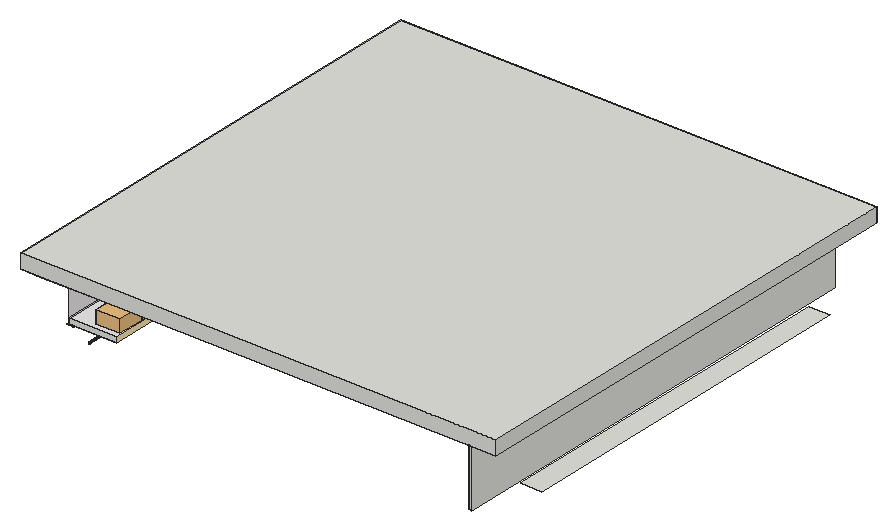
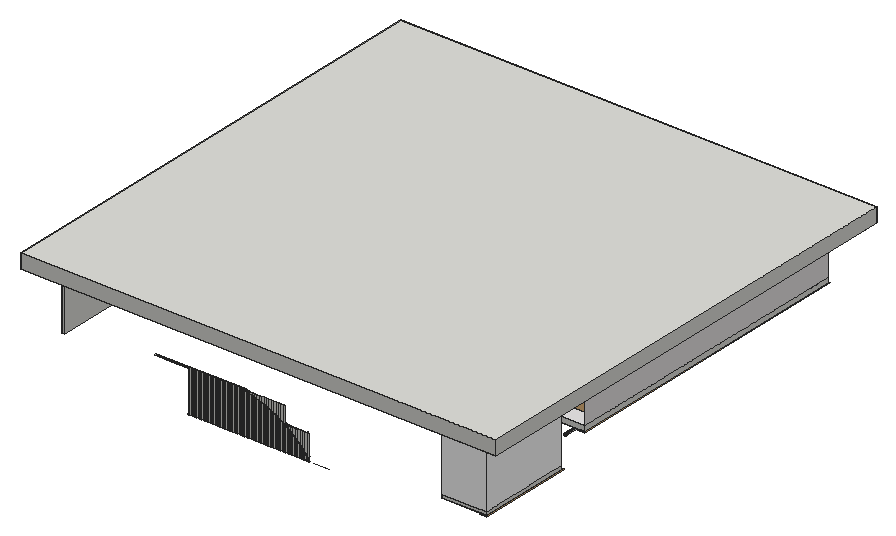
# SketchUp Ruby script. Lengths in inches.
U = 1.inch
M = Sketchup.active_model
def pt(a) = Geom::Point3d.new(a.map { |v| v * U })
def face(e, loops, mat)
  f = e.add_face(loops[0].map { |a| pt(a) })
  loops[1..].each { |l| e.add_face(l.map { |a| pt(a) }).erase! }
  f.material = f.back_material = mat if mat
  f
end
# faces: each face lists its corners as indices into pts; further lists are holes
def faces(e, pts, list, mat = nil) = list.each { |f| face(e, (f[0].is_a?(Array) ? f : [f]).map { |l| l.map { |i| pts[i] } }, mat) }
# xy, xz, yz: faces in a plane at the given z, y or x. An outline is a flat list of corners, or four numbers for a rectangle; further outlines are holes
def ring(l) = l.size == 4 ? [[l[0], l[1]], [l[2], l[1]], [l[2], l[3]], [l[0], l[3]]] : l.each_slice(2).to_a
def flat(e, list, mat, &to3) = list.each { |f| face(e, (f[0].is_a?(Array) ? f : [f]).map { |l| ring(l).map { |u, v| to3.(u, v) } }, mat) }
def xy(e, z, list, mat = nil) = flat(e, list, mat) { |x, y| [x, y, z] }
def xz(e, y, list, mat = nil) = flat(e, list, mat) { |x, z| [x, y, z] }
def yz(e, x, list, mat = nil) = flat(e, list, mat) { |y, z| [x, y, z] }
def lines(e, pts, list) = list.each { |a, b| e.add_line(pt(pts[a]), pt(pts[b])) }
# prism: a flat outline (further loops are holes) pulled along v
def prism(e, loops, v, mat = nil)
  f = face(e, loops, mat); d = Geom::Vector3d.new(v.map { |x| x * U })
  f.pushpull(f.normal.samedirection?(d) ? d.length : -d.length)
end
def box(e, o, s, mat = nil) = prism(e, [[o, [o[0] + s[0], o[1], o[2]], [o[0] + s[0], o[1] + s[1], o[2]], [o[0], o[1] + s[1], o[2]]]], [0, 0, s[2]], mat)
def at(x, y, z, deg = 0) = Geom::Transformation.translation(pt([x, y, z])) * Geom::Transformation.rotation(ORIGIN, Z_AXIS, deg.degrees)
def axes(o, x, y, z) = Geom::Transformation.new([*x, 0, *y, 0, *z, 0, *pt(o).to_a, 1])
def part(name) = M.definitions.add(name)
# library, detail: a bought-in or finely detailed component or shape, given as its bounding box
def library(name, o, s) = part(name).tap { |d| box(d.entities, o, s) }
def detail(e, o, s) = box(e.add_group.entities, o, s)
def put(e, d, t, mat = nil) = e.add_instance(d, t).tap { |i| i.material = mat if mat }
def group(e, t, mat = nil) = e.add_group.tap { |g| g.transformation = t; g.material = mat if mat }.entities
root = M.entities
M.materials.add("Generic").color = [234, 232, 232]
M.materials.add("Gold 10k").color = [251, 232, 180]
M.materials.add("[Color M00]").color = [255, 255, 255]
M.materials.add("[Color M07]").color = [58, 58, 58]
c1 = library("Group\#3",[-0.5,-0.5,-0.1],[3,40,0.2])
c2 = library("Armillary Sphere 37-31",[-7.11,-7.1,0],[14.21,14.18,18.13])
c3 = library("Decorative Deer 209 004",[-1.58,-4.16,0],[3.36,7.25,10.63])
c4 = library("Group\#5",[-0.5,-0.5,-0.1],[3,127.16,0.2])
c5 = library("Clothes 159 005",[-5.11,-5.34,0.03],[10.26,10.67,5.26])
c6 = library("Air Conditioning 001",[-17.62,-7.68,0],[35.24,7.68,11.77])
c7 = library("Fan 90-20",[-15.86,-15.86,-9.19],[31.73,31.72,9.19])
c8 = library("Group\#2",[-0.5,-0.5,-0.1],[3,40,0.2])
c9 = library("Group\#6",[-0.5,-0.5,-0.1],[3,127.16,0.2])
c10 = library("Tlon Light 1950 Ceiling 152 010",[-38.39,-38.39,-3.78],[76.78,76.78,3.41])
c11 = library("Group\#13",[-0.5,-0.5,0],[56.22,1,2.75])
c12 = library("Group\#14",[-0.5,-0.5,0],[1,91.6,2.75])
c13 = library("Group\#15",[-0.5,-0.5,0],[1,91.6,2.75])
c14 = library("Group\#10",[-0.5,-0.5,0],[95.14,130.51,2.5625])
c15 = library("Group\#11",[-0.5,-0.5,0],[127.98,1,2.5625])
c16 = library("Group\#12",[-0.5,-0.5,0],[1,163.35,2.5625])
c17 = library("Group\#16",[-0.5,-0.5,0],[1,164.23,2.5625])
c18 = library("Group\#17",[-0.5,-0.5,0],[127.98,1,2.5625])
xy(root,84.67,[[86.13,189.625,86.28,189.875],[86.875,189.625,87.28,189.875],[87.875,189.625,88.28,189.875],[88.875,189.625,89.28,189.875],[89.875,189.625,90.28,189.875],
  [90.875,189.625,91.28,189.875],[91.875,189.625,92.28,189.875],[92.875,189.625,93.28,189.875],[93.875,189.625,94.28,189.875],[94.875,189.625,95.28,189.875],
  [95.875,189.625,96.28,189.875],[96.875,189.625,97.28,189.875],[97.875,189.625,98.28,189.875],[98.875,189.625,99.28,189.875],[99.875,189.625,100.28,189.875],
  [100.875,189.625,101.28,189.875],[101.875,189.625,102.28,189.875],[102.875,189.625,103.28,189.875],[103.875,189.625,104.28,189.875],[104.875,189.625,105.28,189.875],
  [105.875,189.625,106.28,189.875],[106.875,189.625,107.28,189.875],[107.875,189.625,108.28,189.875],[108.875,189.625,109.28,189.875],[109.875,189.625,110.28,189.875],
  [110.875,189.625,111.28,189.875],[111.875,189.625,112.28,189.875],[112.875,189.625,113.28,189.875],[113.875,189.625,114.28,189.875],[114.875,189.625,115.28,189.875],
  [115.875,189.625,116.28,189.875],[116.875,189.625,117.28,189.875],[117.875,189.625,118.28,189.875],[118.875,189.625,119.28,189.875],[119.875,189.625,120.28,189.875],
  [120.875,189.625,121.28,189.875],[121.875,189.625,122.28,189.875],[122.875,189.625,123.28,189.875],[123.875,189.625,124.28,189.875],[124.875,189.625,125.28,189.875],
  [125.875,189.625,126.28,189.875],[126.875,189.625,127.28,189.875],[127.875,189.625,128.28,189.875],[128.875,189.625,129.28,189.875],[129.875,189.625,130.28,189.875],
  [130.875,189.625,131.28,189.875],[131.875,189.625,132.28,189.875],[132.875,189.625,133.28,189.875],[133.875,189.625,134.28,189.875],[134.28,189.625,134.75,189.875],
  [83.86,189.8125,83.93,189.875],[84.28,189.8125,84.49,189.875],[84.875,189.8125,85.09,189.875],[85.28,189.8125,85.66,189.875],[85.875,189.8125,85.92,189.875],
  [85.92,189.8125,86.04,189.875],[86.04,189.8125,86.13,189.875]])
xy(root,86.88,[[16.5,145.84,33,184.83]])
xy(root,88.09,[[14.5,145.84,33,184.83]],"[Color M00]")
xy(root,96,[[186.625,0,187.95,189],[189,24,198,174]])
xy(root,98.59,[[13.1875,11.43,31,137.59]],"Generic")
xy(root,100.64,[[11.1875,11.43,31,137.59]],"Generic")
xy(root,101.92,[[112.34,189,112.34,189.625,112.875,189.625,112.875,189.875,113.28,189.875,113.28,189.625,113.875,189.625,113.875,189.875,114.28,189.875,114.28,189.625,114.875,189.625,114.875,189.875,115.28,189.875,115.28,189.625,115.875,189.625,115.875,189.875,116.28,189.875,116.28,189.625,116.875,189.625,116.875,189.875,117.28,189.875,117.28,189.625,117.875,189.625,117.875,189.875,118.28,189.875,118.28,189.625,118.875,189.625,118.875,189.875,119.28,189.875,119.28,189.625,119.875,189.625,119.875,189.875,120.28,189.875,120.28,189.625,120.875,189.625,120.875,189.875,121.28,189.875,121.28,189.625,121.875,189.625,121.875,189.875,122.28,189.875,122.28,189.625,122.875,189.625,122.875,189.875,123.28,189.875,123.28,189.625,123.875,189.625,123.875,189.875,124.28,189.875,124.28,189.625,124.875,189.625,124.875,189.875,125.28,189.875,125.28,189.625,125.875,189.625,125.875,189.875,126.28,189.875,126.28,189.625,126.875,189.625,126.875,189.875,127.28,189.875,127.28,189.625,127.875,189.625,127.875,189.875,128.28,189.875,128.28,189.625,128.875,189.625,128.875,189.875,129.28,189.875,129.28,189.625,129.875,189.625,129.875,189.875,130.28,189.875,130.28,189.625,130.875,189.625,130.875,189.875,131.28,189.875,131.28,189.625,131.875,189.625,131.875,189.875,132.28,189.875,132.28,189.625,132.875,189.625,132.875,189.875,133.28,189.875,133.28,189.625,133.875,189.625,133.875,189.875,134.28,189.875,134.28,189.625,134.875,189.625,134.875,189.875,135.28,189.875,135.28,189.75,135.875,189.75,135.875,189.875,136.28,189.875,136.28,189.75,136.875,189.75,136.875,189.875,137.28,189.875,137.28,189.75,137.875,189.75,137.875,189.875,138.28,189.875,138.28,189.75,138.875,189.75,138.875,189.875,139.28,189.875,139.28,189.75,139.875,189.75,139.875,189.875,140.28,189.875,140.28,189.75,140.875,189.75,140.875,189.875,141.28,189.875,141.28,189.75,141.875,189.75,141.875,189.875,142.28,189.875,142.28,189.75,142.875,189.75,142.875,189.875,143.28,189.875,143.28,189.75,143.875,189.75,143.875,189.875,144.28,189.875,144.28,189.75,144.875,189.75,144.875,189.875,145.28,189.875,145.28,189.75,145.875,189.75,145.875,189.875,146.28,189.875,146.28,189.75,146.875,189.75,146.875,189.875,147.28,189.875,147.28,189.75,147.875,189.75,147.875,189.875,148.625,189.875,148.625,189],[134.28,189.625,134.875,189.875],[135.28,189.75,135.875,189.875],[136.28,189.75,136.875,189.875],[137.28,189.75,137.875,189.875],
  [138.28,189.75,138.875,189.875],[139.28,189.75,139.875,189.875],[140.28,189.75,140.875,189.875],[141.28,189.75,141.875,189.875],[142.28,189.75,142.875,189.875],
  [143.28,189.75,143.875,189.875],[144.28,189.75,144.875,189.875],[145.28,189.75,145.875,189.875],[146.28,189.75,146.875,189.875],[147.28,189.75,147.875,189.875]])
xy(root,114.93,[[33,52.82,34.4375,53.82],[34.4375,52.82,34.8125,53.82],[33,95.21,34.4375,96.21],[34.4375,95.21,34.8125,96.21]])
xy(root,114.93,[[33,12.43,34.4375,52.82],[34.4375,12.43,34.8125,52.82],[33,53.82,34.4375,95.21],[34.4375,53.82,34.8125,95.21],[33,96.21,34.4375,136.59],
  [34.4375,96.21,34.8125,136.59]],"[Color M07]")
xy(root,115.83,[[16.5,145.84,33,184.83]])
xy(root,115.93,[[13.1875,11.43,33,137.59]],"Generic")
xy(root,115.93,[[33,11.43,33.4375,12.43],[33.4375,11.43,34.4375,12.43],[34.4375,11.43,34.8125,12.43],[33,12.43,33.4375,136.59],[33.4375,12.43,34.4375,136.59],
  [34.4375,12.43,34.8125,136.59],[33,136.59,33.4375,137.59],[33.4375,136.59,34.4375,137.59],[34.4375,136.59,34.8125,137.59]],"[Color M07]")
xy(root,117.25,[[82.2,49.2,137.43,139.8]])
xy(root,118.7,[[70.35,189,151.87,189.875]])
xy(root,120,[[0,0,0,198,198,198,198,0,189,0,189,189,173.42,189,173.42,190.5,171.08,190.5,171.08,189,153.17,189,153.17,189.875,69.06,189.875,69.06,189,9,189,9,0],[9,0,33,7.36],[[33,0,33,189,69.06,189,69.06,189.875,153.17,189.875,153.17,189,171.08,189,171.08,190.5,173.42,190.5,173.42,189,186.625,189,186.625,0],[46.32,13.32,173.3,176.55]],[186.625,0,187.95,189],[187.95,0,189,189],
  [9,7.36,33,141.67],[9,7.36,33,189],[[62.75,29.75,156.88,159.25],[82.2,49.2,137.43,139.8]],[9,141.67,33,189]])
xy(root,122.5625,[[[46.32,13.32,173.3,176.55],[62.75,29.75,156.88,159.25]]])
xy(root,126,[[0,0,198,198]])
xz(root,0,[[186.625,96,187.95,120],[0,120,198,126]])
xz(root,11.43,[[11.1875,98.59,31,100.64]])
xz(root,12.43,[[33,114.93,34.4375,115.93],[34.4375,114.93,34.8125,115.93]])
xz(root,136.59,[[33,114.93,34.4375,115.93],[34.4375,114.93,34.8125,115.93]])
xz(root,137.59,[[19.57,94.12,19.47,94.13,19.37,94.17,19.29,94.23,19.23,94.32,19.1875,94.41,19.17,94.52,19.1875,94.62,19.23,94.72,19.29,94.8,19.37,94.86,19.47,94.9,19.57,94.92,19.68,94.9,19.77,94.86,19.86,94.8,19.92,94.72,19.96,94.62,19.97,94.52,19.96,94.41,19.92,94.32,19.86,94.23,19.77,94.17,19.68,94.13],[11.1875,98.59,31,100.64]])
xz(root,139.8,[[82.2,117.25,137.43,120]])
xz(root,145.84,[[14.5,86.88,33,88.09],[14.5,88.09,33,115.83]])
xz(root,159.25,[[123.42,120,156.88,122.5625]])
xz(root,184.83,[[14.5,86.88,33,88.09]])
xz(root,184.83,[[14.5,88.09,33,115.83]],"[Color M00]")
xz(root,189,[[186.625,96,187.95,120]])
xz(root,189.625,[[86.28,84.67,86.875,84.67,86.875,88.4,86.28,87.7],[87.28,84.67,87.875,84.67,87.875,89.52,87.68,89.33,87.28,88.86],[88.28,84.67,88.875,84.67,88.875,90.45,88.28,89.89],[89.28,84.67,89.875,84.67,89.875,91.375,89.28,90.82],[90.28,84.67,90.875,84.67,90.875,92.31,90.28,91.75],
  [91.28,84.67,91.875,84.67,91.875,93.09,91.28,92.65],[92.28,84.67,92.875,84.67,92.875,93.84,92.28,93.39],[93.28,84.67,93.875,84.67,93.875,94.58,93.28,94.13],[94.28,84.67,94.875,84.67,94.875,95.32,94.28,94.875],[95.28,84.67,95.875,84.67,95.875,95.91,95.28,95.56],
  [96.28,84.67,96.875,84.67,96.875,96.49,96.28,96.14],[97.28,84.67,97.875,84.67,97.875,97.07,97.28,96.72],[98.28,84.67,98.875,84.67,98.875,97.65,98.28,97.31],[99.28,84.67,99.875,84.67,99.875,98.11,99.28,97.84],[100.28,84.67,100.875,84.67,100.875,98.55,100.28,98.28],
  [101.28,84.67,101.875,84.67,101.875,98.99,101.28,98.73],[102.28,84.67,102.875,84.67,102.875,99.43,102.28,99.17],[103.28,84.67,103.875,84.67,103.875,99.8,103.28,99.61],[104.28,84.67,104.875,84.67,104.875,100.11,104.28,99.92],[105.28,84.67,105.875,84.67,105.875,100.43,105.28,100.24],
  [106.28,84.67,106.875,84.67,106.875,100.74,106.28,100.55],[107.28,84.67,107.875,84.67,107.875,101.04,107.73,101.01,107.28,100.87],[108.28,84.67,108.875,84.67,108.875,101.24,108.28,101.12],[109.28,84.67,109.875,84.67,109.875,101.44,109.28,101.32],[110.28,84.67,110.875,84.67,110.875,101.63,110.28,101.51],
  [111.28,84.67,111.875,84.67,111.875,101.83,111.28,101.71],[112.28,84.67,112.875,84.67,112.875,101.92,112.34,101.92,112.28,101.91],[113.28,84.67,113.875,101.92],[114.28,84.67,114.875,101.92],[115.28,84.67,115.875,101.92],
  [116.28,84.67,116.875,101.92],[117.28,84.67,117.875,101.92],[118.28,84.67,118.875,101.92],[119.28,84.67,119.875,101.92],[120.28,84.67,120.875,101.92],
  [121.28,84.67,121.875,101.92],[122.28,84.67,122.875,101.92],[123.28,84.67,123.875,101.92],[124.28,84.67,124.875,101.92],[125.28,84.67,125.875,101.92],
  [126.28,84.67,126.875,101.92],[127.28,84.67,127.875,101.92],[128.28,84.67,128.875,101.92],[129.28,84.67,129.875,101.92],[130.28,84.67,130.875,101.92],
  [131.28,84.67,131.875,101.92],[132.28,84.67,132.875,101.92],[133.28,84.67,133.875,101.92]])
xz(root,189.875,[[85.875,84.67,86.28,84.67,86.28,87.7,85.875,87.24],[86.875,84.67,87.28,84.67,87.28,88.86,86.875,88.4],[87.875,84.67,88.28,84.67,88.28,89.89,87.875,89.52],[88.875,84.67,89.28,84.67,89.28,90.82,88.875,90.45],[89.875,84.67,90.28,84.67,90.28,91.75,89.875,91.375],
  [90.875,84.67,91.28,84.67,91.28,92.65,91.12,92.53,90.875,92.31],[91.875,84.67,92.28,84.67,92.28,93.39,91.875,93.09],[92.875,84.67,93.28,84.67,93.28,94.13,92.875,93.84],[93.875,84.67,94.28,84.67,94.28,94.875,93.875,94.58],[94.875,84.67,95.28,84.67,95.28,95.56,94.89,95.33,94.875,95.32],
  [95.875,84.67,96.28,84.67,96.28,96.14,95.875,95.91],[96.875,84.67,97.28,84.67,97.28,96.72,96.875,96.49],[97.875,84.67,98.28,84.67,98.28,97.31,97.875,97.07],[98.875,84.67,99.28,84.67,99.28,97.84,98.95,97.7,98.875,97.65],[99.875,84.67,100.28,84.67,100.28,98.28,99.875,98.11],
  [100.875,84.67,101.28,84.67,101.28,98.73,100.875,98.55],[101.875,84.67,102.28,84.67,102.28,99.17,101.875,98.99],[102.875,84.67,103.28,84.67,103.28,99.61,103.25,99.6,102.875,99.43],[103.875,84.67,104.28,84.67,104.28,99.92,103.875,99.8],[104.875,84.67,105.28,84.67,105.28,100.24,104.875,100.11],
  [105.875,84.67,106.28,84.67,106.28,100.55,105.875,100.43],[106.875,84.67,107.28,84.67,107.28,100.87,106.875,100.74],[107.875,84.67,108.28,84.67,108.28,101.12,107.875,101.04],[108.875,84.67,109.28,84.67,109.28,101.32,108.875,101.24],[109.875,84.67,110.28,84.67,110.28,101.51,109.875,101.44],
  [110.875,84.67,111.28,84.67,111.28,101.71,110.875,101.63],[111.875,84.67,112.28,84.67,112.28,101.91,111.875,101.83],[112.875,84.67,113.28,101.92],[113.875,84.67,114.28,101.92],[114.875,84.67,115.28,101.92],
  [115.875,84.67,116.28,101.92],[116.875,84.67,117.28,101.92],[117.875,84.67,118.28,101.92],[118.875,84.67,119.28,101.92],[119.875,84.67,120.28,101.92],
  [120.875,84.67,121.28,101.92],[121.875,84.67,122.28,101.92],[122.875,84.67,123.28,101.92],[123.875,84.67,124.28,101.92],[124.875,84.67,125.28,101.92],
  [125.875,84.67,126.28,101.92],[126.875,84.67,127.28,101.92],[127.875,84.67,128.28,101.92],[128.875,84.67,129.28,101.92],[129.875,84.67,130.28,101.92],
  [130.875,84.67,131.28,101.92],[131.875,84.67,132.28,101.92],[132.875,84.67,133.28,101.92],[133.875,84.67,134.28,101.92],[84.28,85.28,84.62,85.77,84.875,86.07,84.875,95.32,84.28,94.875],
  [85.28,86.54,85.875,87.24,85.875,95.32,85.28,94.875],[86.28,87.7,86.875,88.4,86.875,95.32,86.28,94.875],[87.28,88.86,87.68,89.33,87.875,89.52,87.875,95.32,87.28,94.875],[88.28,89.89,88.875,90.45,88.875,95.32,88.28,94.875],[89.28,90.82,89.875,91.375,89.875,95.32,89.28,94.875],
  [90.28,91.75,90.875,92.31,90.875,95.32,90.28,94.875],[91.28,92.65,91.875,93.09,91.875,95.32,91.28,94.875],[92.28,93.39,92.875,93.84,92.875,95.32,92.28,94.875],[93.28,94.13,93.875,94.58,93.875,95.32,93.28,94.875],[94.28,94.875,94.875,95.32,94.875,101.92,94.28,101.92],
  [95.28,95.56,95.875,95.91,95.875,101.92,95.28,101.92],[96.28,96.14,96.875,96.49,96.875,101.92,96.28,101.92],[97.28,96.72,97.875,97.07,97.875,101.92,97.28,101.92],[98.28,97.31,98.875,97.65,98.875,101.92,98.28,101.92],[99.28,97.84,99.875,98.11,99.875,101.92,99.28,101.92],
  [100.28,98.28,100.875,98.55,100.875,101.92,100.28,101.92],[101.28,98.73,101.875,98.99,101.875,101.92,101.28,101.92],[102.28,99.17,102.875,99.43,102.875,101.92,102.28,101.92],[103.28,99.61,103.875,99.8,103.875,101.92,103.28,101.92],[104.28,99.92,104.875,100.11,104.875,101.92,104.28,101.92],
  [105.28,100.24,105.875,100.43,105.875,101.92,105.28,101.92],[106.28,100.55,106.875,100.74,106.875,101.92,106.28,101.92],[107.28,100.87,107.73,101.01,107.875,101.04,107.875,101.92,107.28,101.92],[108.28,101.12,108.875,101.24,108.875,101.92,108.28,101.92],[109.28,101.32,109.875,101.44,109.875,101.92,109.28,101.92],
  [110.28,101.51,110.875,101.63,110.875,101.92,110.28,101.92],[111.28,101.71,111.875,101.83,111.875,101.92,111.28,101.92],[112.28,101.91,112.34,101.92,112.28,101.92]])
xz(root,198,[[0,120,198,126]])
yz(root,0,[[0,120,198,126]])
yz(root,11.1875,[[11.43,98.59,137.59,100.64]])
yz(root,11.1875,[[11.43,100.64,137.59,115.93]],"Generic")
yz(root,14.5,[[145.84,86.88,184.83,88.09]])
yz(root,14.5,[[145.84,88.09,184.83,115.83]],"[Color M00]")
yz(root,31,[[11.43,98.59,137.59,100.64]],"Gold 10k")
yz(root,33,[[145.84,86.88,184.83,88.09]])
yz(root,33,[[12.43,114.93,136.59,115.93]],"[Color M07]")
yz(root,34.4375,[[12.43,114.93,136.59,115.93]])
yz(root,34.8125,[[12.43,114.93,136.59,115.93]],"[Color M07]")
yz(root,84.28,[[189.8125,84.67,189.875,85.28]])
yz(root,84.875,[[189.8125,84.67,189.875,86.07]])
yz(root,85.28,[[189.8125,84.67,189.875,86.54]])
yz(root,85.875,[[189.8125,84.67,189.875,87.24]])
yz(root,86.28,[[189.625,84.67,189.875,87.7]])
yz(root,86.875,[[189.625,84.67,189.875,88.4]])
yz(root,87.28,[[189.625,84.67,189.875,88.86]])
yz(root,87.875,[[189.625,84.67,189.875,89.52]])
yz(root,88.28,[[189.625,84.67,189.875,89.89]])
yz(root,88.875,[[189.625,84.67,189.875,90.45]])
yz(root,89.28,[[189.625,84.67,189.875,90.82]])
yz(root,89.875,[[189.625,84.67,189.875,91.375]])
yz(root,90.28,[[189.625,84.67,189.875,91.75]])
yz(root,90.875,[[189.625,84.67,189.875,92.31]])
yz(root,91.28,[[189.625,84.67,189.875,92.65]])
yz(root,91.875,[[189.625,84.67,189.875,93.09]])
yz(root,92.28,[[189.625,84.67,189.875,93.39]])
yz(root,92.875,[[189.625,84.67,189.875,93.84]])
yz(root,93.28,[[189.625,84.67,189.875,94.13]])
yz(root,93.875,[[189.625,84.67,189.875,94.58]])
yz(root,94.28,[[189.625,84.67,189.875,94.875]])
yz(root,94.875,[[189.625,84.67,189.875,95.32]])
yz(root,95.28,[[189.625,84.67,189.875,95.56]])
yz(root,95.875,[[189.625,84.67,189.875,95.91]])
yz(root,96.28,[[189.625,84.67,189.875,96.14]])
yz(root,96.875,[[189.625,84.67,189.875,96.49]])
yz(root,97.28,[[189.625,84.67,189.875,96.72]])
yz(root,97.875,[[189.625,84.67,189.875,97.07]])
yz(root,98.28,[[189.625,84.67,189.875,97.31]])
yz(root,98.875,[[189.625,84.67,189.875,97.65]])
yz(root,99.28,[[189.625,84.67,189.875,97.84]])
yz(root,99.875,[[189.625,84.67,189.875,98.11]])
yz(root,100.28,[[189.625,84.67,189.875,98.28]])
yz(root,100.875,[[189.625,84.67,189.875,98.55]])
yz(root,101.28,[[189.625,84.67,189.875,98.73]])
yz(root,101.875,[[189.625,84.67,189.875,98.99]])
yz(root,102.28,[[189.625,84.67,189.875,99.17]])
yz(root,102.875,[[189.625,84.67,189.875,99.43]])
yz(root,103.28,[[189.625,84.67,189.875,99.61]])
yz(root,103.875,[[189.625,84.67,189.875,99.8]])
yz(root,104.28,[[189.625,84.67,189.875,99.92]])
yz(root,104.875,[[189.625,84.67,189.875,100.11]])
yz(root,105.28,[[189.625,84.67,189.875,100.24]])
yz(root,105.875,[[189.625,84.67,189.875,100.43]])
yz(root,106.28,[[189.625,84.67,189.875,100.55]])
yz(root,106.875,[[189.625,84.67,189.875,100.74]])
yz(root,107.28,[[189.625,84.67,189.875,100.87]])
yz(root,107.875,[[189.625,84.67,189.875,101.04]])
yz(root,108.28,[[189.625,84.67,189.875,101.12]])
yz(root,108.875,[[189.625,84.67,189.875,101.24]])
yz(root,109.28,[[189.625,84.67,189.875,101.32]])
yz(root,109.875,[[189.625,84.67,189.875,101.44]])
yz(root,110.28,[[189.625,84.67,189.875,101.51]])
yz(root,110.875,[[189.625,84.67,189.875,101.63]])
yz(root,111.28,[[189.625,84.67,189.875,101.71]])
yz(root,111.875,[[189.625,84.67,189.875,101.83]])
yz(root,112.28,[[189.625,84.67,189.875,101.91]])
yz(root,112.875,[[189.625,84.67,189.875,101.92]])
yz(root,113.28,[[189.625,84.67,189.875,101.92]])
yz(root,113.875,[[189.625,84.67,189.875,101.92]])
yz(root,114.28,[[189.625,84.67,189.875,101.92]])
yz(root,114.875,[[189.625,84.67,189.875,101.92]])
yz(root,115.28,[[189.625,84.67,189.875,101.92]])
yz(root,115.875,[[189.625,84.67,189.875,101.92]])
yz(root,116.28,[[189.625,84.67,189.875,101.92]])
yz(root,116.875,[[189.625,84.67,189.875,101.92]])
yz(root,117.28,[[189.625,84.67,189.875,101.92]])
yz(root,117.875,[[189.625,84.67,189.875,101.92]])
yz(root,118.28,[[189.625,84.67,189.875,101.92]])
yz(root,118.875,[[189.625,84.67,189.875,101.92]])
yz(root,119.28,[[189.625,84.67,189.875,101.92]])
yz(root,119.875,[[189.625,84.67,189.875,101.92]])
yz(root,120.28,[[189.625,84.67,189.875,101.92]])
yz(root,120.875,[[189.625,84.67,189.875,101.92]])
yz(root,121.28,[[189.625,84.67,189.875,101.92]])
yz(root,121.875,[[189.625,84.67,189.875,101.92]])
yz(root,122.28,[[189.625,84.67,189.875,101.92]])
yz(root,122.875,[[189.625,84.67,189.875,101.92]])
yz(root,123.28,[[189.625,84.67,189.875,101.92]])
yz(root,123.875,[[189.625,84.67,189.875,101.92]])
yz(root,124.28,[[189.625,84.67,189.875,101.92]])
yz(root,124.875,[[189.625,84.67,189.875,101.92]])
yz(root,125.28,[[189.625,84.67,189.875,101.92]])
yz(root,125.875,[[189.625,84.67,189.875,101.92]])
yz(root,126.28,[[189.625,84.67,189.875,101.92]])
yz(root,126.875,[[189.625,84.67,189.875,101.92]])
yz(root,127.28,[[189.625,84.67,189.875,101.92]])
yz(root,127.875,[[189.625,84.67,189.875,101.92]])
yz(root,128.28,[[189.625,84.67,189.875,101.92]])
yz(root,128.875,[[189.625,84.67,189.875,101.92]])
yz(root,129.28,[[189.625,84.67,189.875,101.92]])
yz(root,129.875,[[189.625,84.67,189.875,101.92]])
yz(root,130.28,[[189.625,84.67,189.875,101.92]])
yz(root,130.875,[[189.625,84.67,189.875,101.92]])
yz(root,131.28,[[189.625,84.67,189.875,101.92]])
yz(root,131.875,[[189.625,84.67,189.875,101.92]])
yz(root,132.28,[[189.625,84.67,189.875,101.92]])
yz(root,132.875,[[189.625,84.67,189.875,101.92]])
yz(root,133.28,[[189.625,84.67,189.875,101.92]])
yz(root,133.875,[[189.625,84.67,189.875,101.92]])
yz(root,134.28,[[189.625,84.67,189.875,101.92]])
yz(root,186.625,[[0,96,189,120]])
yz(root,187.95,[[0,96,189,120]])
yz(root,198,[[0,120,198,126]])
p = [[84.28,189.875,85.28],[84.62,189.875,85.77],[84.62,189.8125,85.77],[84.28,189.8125,85.28],[87.68,189,89.33],[84.62,189,85.77],
  [84.875,189.8125,86.07],[84.875,189.875,86.07],[85.28,189.875,86.54],[85.28,189.8125,86.54],[85.875,189.8125,87.24],[85.875,189.875,87.24],
  [86.28,189.875,87.7],[86.28,189.625,87.7],[86.875,189.625,88.4],[86.875,189.875,88.4],[87.28,189.875,88.86],[87.28,189.625,88.86],
  [87.68,189.625,89.33],[87.68,189.875,89.33],[91.12,189,92.53],[87.875,189.625,89.52],[87.875,189.875,89.52],[88.28,189.875,89.89],
  [88.28,189.625,89.89],[88.875,189.625,90.45],[88.875,189.875,90.45],[89.28,189.875,90.82],[89.28,189.625,90.82],[89.875,189.625,91.375],
  [89.875,189.875,91.375],[90.28,189.875,91.75],[90.28,189.625,91.75],[90.875,189.625,92.31],[90.875,189.875,92.31],[91.12,189.875,92.53],
  [94.89,189,95.33],[91.28,189.875,92.65],[91.28,189.625,92.65],[91.875,189.625,93.09],[91.875,189.875,93.09],[92.28,189.875,93.39],
  [92.28,189.625,93.39],[92.875,189.625,93.84],[92.875,189.875,93.84],[93.28,189.875,94.13],[93.28,189.625,94.13],[93.875,189.625,94.58],
  [93.875,189.875,94.58],[94.28,189.875,94.875],[94.28,189.625,94.875],[94.875,189.625,95.32],[94.875,189.875,95.32],[94.89,189.875,95.33],
  [19.37,137.59,94.17],[19.47,137.59,94.13],[19.47,11.43,94.13],[19.37,11.43,94.17],[19.57,137.59,94.12],[19.57,11.43,94.12],
  [19.68,137.59,94.13],[19.68,11.43,94.13],[19.77,137.59,94.17],[19.77,11.43,94.17],[19.23,137.59,94.32],[19.29,137.59,94.23],
  [19.29,11.43,94.23],[19.23,11.43,94.32],[19.86,137.59,94.23],[19.86,11.43,94.23],[19.92,137.59,94.32],[19.92,11.43,94.32],
  [19.1875,137.59,94.41],[19.1875,11.43,94.41],[19.96,137.59,94.41],[19.96,11.43,94.41],[19.17,137.59,94.52],[19.17,11.43,94.52],
  [19.97,137.59,94.52],[19.97,11.43,94.52],[19.1875,137.59,94.62],[19.1875,11.43,94.62],[19.96,137.59,94.62],[19.96,11.43,94.62],
  [19.23,137.59,94.72],[19.23,11.43,94.72],[19.92,137.59,94.72],[19.92,11.43,94.72],[19.29,137.59,94.8],[19.29,11.43,94.8],
  [19.86,137.59,94.8],[19.86,11.43,94.8],[19.37,137.59,94.86],[19.37,11.43,94.86],[19.77,137.59,94.86],[19.77,11.43,94.86],
  [19.47,137.59,94.9],[19.47,11.43,94.9],[19.57,137.59,94.92],[19.57,11.43,94.92],[19.68,137.59,94.9],[19.68,11.43,94.9],
  [98.95,189,97.7],[95.28,189.875,95.56],[95.28,189.625,95.56],[95.875,189.625,95.91],[95.875,189.875,95.91],[96.28,189.875,96.14],
  [96.28,189.625,96.14],[96.875,189.625,96.49],[96.875,189.875,96.49],[97.28,189.875,96.72],[97.28,189.625,96.72],[97.875,189.625,97.07],
  [97.875,189.875,97.07],[98.28,189.875,97.31],[98.28,189.625,97.31],[98.875,189.625,97.65],[98.875,189.875,97.65],[98.95,189.875,97.7],
  [103.25,189,99.6],[99.28,189.875,97.84],[99.28,189.625,97.84],[99.875,189.625,98.11],[99.875,189.875,98.11],[100.28,189.875,98.28],
  [100.28,189.625,98.28],[100.875,189.625,98.55],[100.875,189.875,98.55],[101.28,189.875,98.73],[101.28,189.625,98.73],[101.875,189.625,98.99],
  [101.875,189.875,98.99],[102.28,189.875,99.17],[102.28,189.625,99.17],[102.875,189.625,99.43],[102.875,189.875,99.43],[103.25,189.875,99.6],
  [107.73,189,101.01],[103.28,189.875,99.61],[103.28,189.625,99.61],[103.875,189.625,99.8],[103.875,189.875,99.8],[104.28,189.875,99.92],
  [104.28,189.625,99.92],[104.875,189.625,100.11],[104.875,189.875,100.11],[105.28,189.875,100.24],[105.28,189.625,100.24],[105.875,189.625,100.43],
  [105.875,189.875,100.43],[106.28,189.875,100.55],[106.28,189.625,100.55],[106.875,189.625,100.74],[106.875,189.875,100.74],[107.28,189.875,100.87],
  [107.28,189.625,100.87],[107.73,189.625,101.01],[107.73,189.875,101.01],[112.34,189,101.92],[107.875,189.625,101.04],[107.875,189.875,101.04],
  [108.28,189.875,101.12],[108.28,189.625,101.12],[108.875,189.625,101.24],[108.875,189.875,101.24],[109.28,189.875,101.32],[109.28,189.625,101.32],
  [109.875,189.625,101.44],[109.875,189.875,101.44],[110.28,189.875,101.51],[110.28,189.625,101.51],[110.875,189.625,101.63],[110.875,189.875,101.63],
  [111.28,189.875,101.71],[111.28,189.625,101.71],[111.875,189.625,101.83],[111.875,189.875,101.83],[112.28,189.875,101.91],[112.28,189.625,101.91],
  [112.34,189.625,101.92],[112.34,189.875,101.92],[82.43,189.875,84.67],[82.55,189.875,84.67],[82.7,189.875,84.67],[82.17,189.875,84.67],
  [81.26,189.875,84.67],[81.38,189.875,84.67],[81.53,189.875,84.67],[81.6,189.875,84.67],[81,189.875,84.67],[80.38,189.875,84.67],
  [80.53,189.875,84.67],[80,189.875,84.67],[80.26,189.875,84.67],[80.6,189.875,84.67],[79.26,189.875,84.67],[79.38,189.875,84.67],
  [79.53,189.875,84.67],[79,189.875,84.67],[79.6,189.875,84.67],[78.26,189.875,84.67],[78.38,189.875,84.67],[78,189.875,84.67],
  [78.53,189.875,84.67],[78.6,189.875,84.67],[77.26,189.875,84.67],[77.38,189.875,84.67],[77,189.875,84.67],[77.53,189.875,84.67],
  [77.6,189.875,84.67],[76.38,189.875,84.67],[76.53,189.875,84.67],[76.6,189.875,84.67],[76,189.875,84.67],[76.26,189.875,84.67]]
faces(root,p,[[0,1,2,3],[4,5,2,6,7,8,9,10,11,12,13,14,15,16,17,18],[1,7,6,2],[8,11,10,9],[12,15,14,13],[16,19,18,17],[20,4,18,21,22,23,24,25,26,27,28,29,30,31,32,33,34,35],[19,22,21,18],
  [23,26,25,24],[27,30,29,28],[31,34,33,32],[36,20,35,37,38,39,40,41,42,43,44,45,46,47,48,49,50,51,52,53],[37,40,39,38],[41,44,43,42],[45,48,47,46],[49,52,51,50],
  [102,36,53,103,104,105,106,107,108,109,110,111,112,113,114,115,116,117,118,119],[103,106,105,104],[107,110,109,108],[111,114,113,112],[115,118,117,116],[120,102,119,121,122,123,124,125,126,127,128,129,130,131,132,133,134,135,136,137],[121,124,123,122],[125,128,127,126],
  [129,132,131,130],[133,136,135,134],[138,120,137,139,140,141,142,143,144,145,146,147,148,149,150,151,152,153,154,155,156,157],[139,142,141,140],[143,146,145,144],[147,150,149,148],[151,154,153,152],[155,158,157,156],
  [159,138,157,160,161,162,163,164,165,166,167,168,169,170,171,172,173,174,175,176,177,178,179,180],[158,161,160,157],[162,165,164,163],[166,169,168,167],[170,173,172,171],[174,177,176,175],[178,181,180,179]])
faces(root,p,[[54,55,56,57],[55,58,59,56],[58,60,61,59],[60,62,63,61],[64,65,66,67],[65,54,57,66],[62,68,69,63],[68,70,71,69],
  [72,64,67,73],[70,74,75,71],[76,72,73,77],[74,78,79,75],[80,76,77,81],[78,82,83,79],[84,80,81,85],[82,86,87,83],
  [88,84,85,89],[86,90,91,87],[92,88,89,93],[90,94,95,91],[96,92,93,97],[98,96,97,99],[100,98,99,101],[94,100,101,95]],"Generic")
lines(root,p,[[182,183],[183,184],[185,182],[186,187],[188,189],[187,188],[190,186],[191,192],[193,194],[192,195],[194,191],[196,197],
  [197,198],[199,196],[198,200],[201,202],[203,201],[202,204],[204,205],[206,207],[208,206],[207,209],[209,210],[211,212],
  [212,213],[214,215],[215,211]])
put(root,c1,at(14.5,145.84,86.88))
put(root,c2,at(25.875,170.06,88.09))
put(root,c3,axes([27.08,156.5625,88.09],[0,1.4338,0],[-1.4338,0,0],[0,0,1.4338]))
put(root,c4,at(11.1875,11.43,98.59))
put(root,c5,at(25.2,19.27,100.64))
put(root,c5,at(25.24,30.875,100.64))
put(root,c5,at(25.4375,44.03,100.64))
put(root,c5,at(25.09,57.41,100.64))
put(root,c5,at(23.83,71.42,100.64))
put(root,c5,at(23.41,84.6,100.64))
put(root,c5,at(23.53,97.58,100.64))
put(root,c5,at(21.71,111.51,100.64))
put(root,c5,at(18.66,125.07,100.64))
put(root,c6,at(186.625,98.42,106.61,-90))
put(root,c7,at(103.83,85.63,117.25))
put(root,c8,at(14.5,145.84,115.83))
put(root,c9,at(11.1875,11.43,115.93))
put(root,c10,axes([87.01,56.04,117.35],[0.0494,0,0],[0,0.0494,0],[0,0,0.0494]))
put(root,c10,axes([87.01,70.54,117.35],[0.0494,0,0],[0,0.0494,0],[0,0,0.0494]))
put(root,c10,axes([87.01,85.04,117.35],[0.0494,0,0],[0,0.0494,0],[0,0,0.0494]))
put(root,c10,axes([87.01,99.54,117.35],[0.0494,0,0],[0,0.0494,0],[0,0,0.0494]))
put(root,c10,axes([87.01,114.04,117.35],[0.0494,0,0],[0,0.0494,0],[0,0,0.0494]))
put(root,c10,axes([126.51,56.04,117.35],[0.0494,0,0],[0,0.0494,0],[0,0,0.0494]))
put(root,c10,axes([126.51,70.42,117.35],[0.0494,0,0],[0,0.0494,0],[0,0,0.0494]))
put(root,c10,axes([126.51,84.79,117.35],[0.0494,0,0],[0,0.0494,0],[0,0,0.0494]))
put(root,c10,axes([126.51,99.17,117.35],[0.0494,0,0],[0,0.0494,0],[0,0,0.0494]))
put(root,c10,axes([126.51,113.54,117.35],[0.0494,0,0],[0,0.0494,0],[0,0,0.0494]))
put(root,c11,at(82.2,49.2,117.25))
put(root,c12,at(137.43,49.2,117.25))
put(root,c13,at(82.2,49.2,117.25))
put(root,c10,axes([178.39,11.24,120.1],[0.0494,0,0],[0,0.0494,0],[0,0,0.0494]))
put(root,c10,axes([178.39,168.12,120.1],[0.0494,0,0],[0,0.0494,0],[0,0,0.0494]))
put(root,c10,axes([42.13,168.12,120.1],[0.0494,0,0],[0,0.0494,0],[0,0,0.0494]))
put(root,c10,axes([42.13,11.93,120.1],[0.0494,0,0],[0,0.0494,0],[0,0,0.0494]))
put(root,c14,at(62.75,29.75,120))
put(root,c15,at(46.32,13.32,120))
put(root,c16,at(173.3,13.32,120))
put(root,c17,at(46.32,13.32,120))
put(root,c18,at(46.32,176.55,120))
